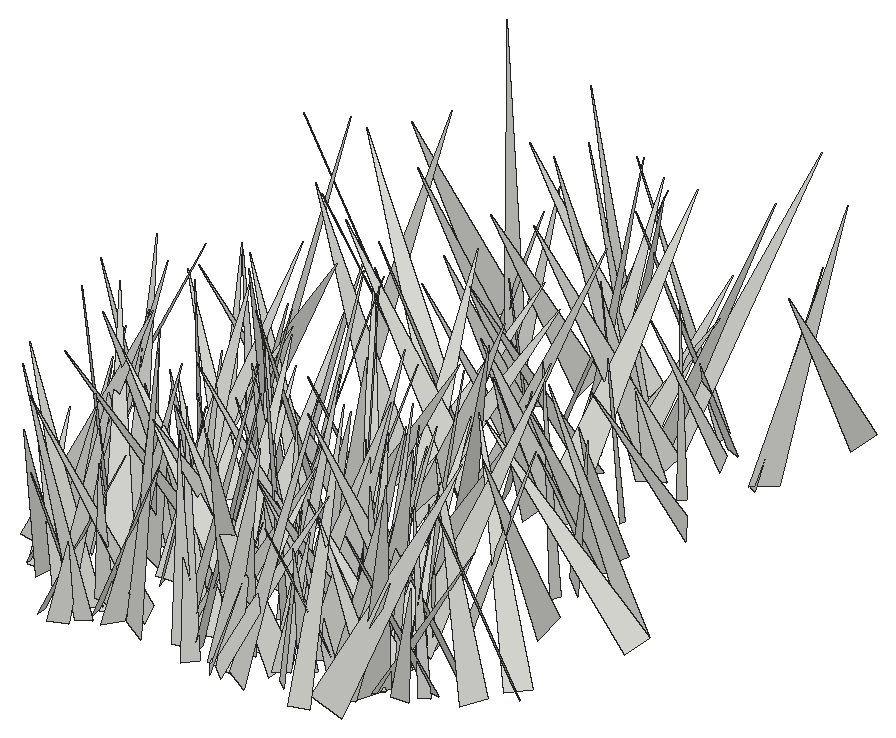
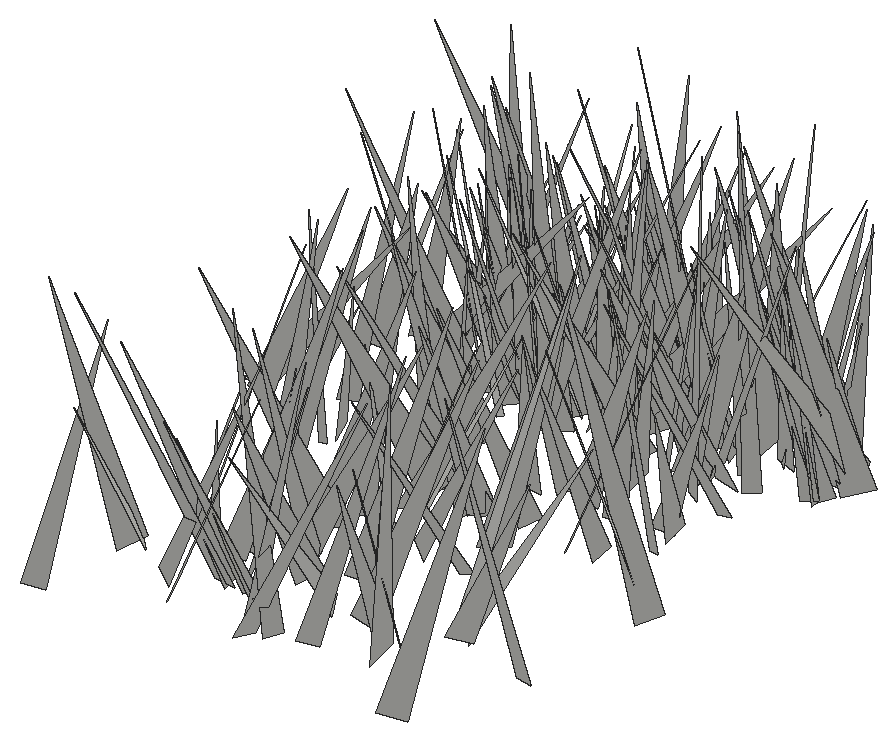
# SketchUp Ruby script. Lengths in inches.
U = 1.inch
M = Sketchup.active_model
def pt(a) = Geom::Point3d.new(a.map { |v| v * U })
def face(e, loops, mat)
  f = e.add_face(loops[0].map { |a| pt(a) })
  loops[1..].each { |l| e.add_face(l.map { |a| pt(a) }).erase! }
  f.material = f.back_material = mat if mat
  f
end
# faces: each face lists its corners as indices into pts; further lists are holes
def faces(e, pts, list, mat = nil) = list.each { |f| face(e, (f[0].is_a?(Array) ? f : [f]).map { |l| l.map { |i| pts[i] } }, mat) }
# xy, xz, yz: faces in a plane at the given z, y or x. An outline is a flat list of corners, or four numbers for a rectangle; further outlines are holes
def ring(l) = l.size == 4 ? [[l[0], l[1]], [l[2], l[1]], [l[2], l[3]], [l[0], l[3]]] : l.each_slice(2).to_a
def flat(e, list, mat, &to3) = list.each { |f| face(e, (f[0].is_a?(Array) ? f : [f]).map { |l| ring(l).map { |u, v| to3.(u, v) } }, mat) }
def xy(e, z, list, mat = nil) = flat(e, list, mat) { |x, y| [x, y, z] }
def xz(e, y, list, mat = nil) = flat(e, list, mat) { |x, z| [x, y, z] }
def yz(e, x, list, mat = nil) = flat(e, list, mat) { |y, z| [x, y, z] }
def lines(e, pts, list) = list.each { |a, b| e.add_line(pt(pts[a]), pt(pts[b])) }
# prism: a flat outline (further loops are holes) pulled along v
def prism(e, loops, v, mat = nil)
  f = face(e, loops, mat); d = Geom::Vector3d.new(v.map { |x| x * U })
  f.pushpull(f.normal.samedirection?(d) ? d.length : -d.length)
end
def box(e, o, s, mat = nil) = prism(e, [[o, [o[0] + s[0], o[1], o[2]], [o[0] + s[0], o[1] + s[1], o[2]], [o[0], o[1] + s[1], o[2]]]], [0, 0, s[2]], mat)
def at(x, y, z, deg = 0) = Geom::Transformation.translation(pt([x, y, z])) * Geom::Transformation.rotation(ORIGIN, Z_AXIS, deg.degrees)
def axes(o, x, y, z) = Geom::Transformation.new([*x, 0, *y, 0, *z, 0, *pt(o).to_a, 1])
def part(name) = M.definitions.add(name)
# library, detail: a bought-in or finely detailed component or shape, given as its bounding box
def library(name, o, s) = part(name).tap { |d| box(d.entities, o, s) }
def detail(e, o, s) = box(e.add_group.entities, o, s)
def put(e, d, t, mat = nil) = e.add_instance(d, t).tap { |i| i.material = mat if mat }
def group(e, t, mat = nil) = e.add_group.tap { |g| g.transformation = t; g.material = mat if mat }.entities
root = M.entities
c1 = part("fur_instance\#9")
p = [[0.8125,0,1.79],[0.67,-0.02,1.48],[0,-0.11,0],[0,0.11,0]]
faces(c1.entities,p,[[0,1,2,3]])
put(root,c1,axes([514.54,139.38,-21.86],[4.00541,-4.88826,1.49079],[-5.10449,-3.91872,0.86522],[-0.24835,1.7057,6.26017]))
put(root,c1,axes([507.39,138.36,-21.66],[-2.16703,-5.16397,2.37315],[-5.48971,1.24499,-2.30381],[-1.47021,2.96275,5.10441]))
put(root,c1,axes([505.36,140.28,-21.86],[-1.78915,-3.44674,0.35763],[-3.41457,1.82215,0.479],[0.59044,0.09337,3.85378]))
put(root,c1,axes([503.11,141.12,-21.86],[4.81338,-2.70132,0.36004],[-2.51999,-4.69011,-1.49931],[-1.0375,-1.14068,5.31205]))
put(root,c1,axes([509.17,140.8,-21.86],[-5.82237,-2.50943,0.01956],[-2.48564,5.77362,0.82736],[0.34528,-0.75212,6.28591]))
put(root,c1,axes([514.33,138.67,-21.86],[3.35941,2.47012,0.56366],[2.52325,-3.34641,-0.37364],[-0.22894,-0.63632,4.15301]))
put(root,c1,axes([507.27,139.99,-21.86],[1.42662,-4.11071,0.89066],[-4.20545,-1.41051,0.22612],[-0.07357,0.91596,4.34535]))
put(root,c1,axes([512.17,139.48,-21.86],[-0.91503,4.79321,2.31879],[5.31141,0.98733,0.05504],[0.37492,-2.28894,4.87946]))
put(root,c1,axes([513.125,142.4375,-21.86],[6.38764,-4.10189,0.26345],[-3.90919,-6.21298,-1.95294],[-1.27011,-1.50671,7.33577]))
put(root,c1,axes([505.22,138.04,-21.86],[4.04294,1.47662,0.10602],[1.40514,-3.92456,1.07725],[-0.46609,0.97696,4.16717]))
put(root,c1,axes([514.49,138.9,-21.86],[3.25743,4.86298,0.41292],[4.6269,-2.91916,-2.12138],[1.55271,-1.50328,5.4552]))
put(root,c1,axes([514.69,140.74,-21.86],[1.67883,-4.20753,0.33675],[-4.18563,-1.61266,0.71764],[0.54516,0.57551,4.47289]))
put(root,c1,axes([516.81,140.66,-21.86],[-6.87538,0.87455,0.95023],[1.06547,6.75006,1.49673],[0.72976,-1.61573,6.76724]))
put(root,c1,axes([507.15,139.64,-21.86],[4.62251,0.92588,0.22465],[0.9419,-4.60847,-0.38752],[-0.14333,-0.42437,4.69837]))
put(root,c1,axes([506.65,139.62,-21.86],[0.94645,-5.69848,3.07489],[-6.04954,-1.88624,-1.63358],[-2.30884,2.60631,5.54074]))
put(root,c1,axes([521.48,141.45,-21.86],[6.44633,-3.37101,0.63256],[-3.2949,-6.46051,-0.8512],[-0.95262,-0.46602,7.22457]))
put(root,c1,axes([509.54,139.25,-21.86],[3.62939,6.32437,2.66269],[6.74766,-3.83695,-0.08396],[-1.24771,-2.35377,7.2913]))
put(root,c1,axes([511.83,140,-21.66],[6.05057,5.41917,1.99571],[5.77348,-5.74186,-1.9125],[-0.1309,-2.76104,7.89425]))
put(root,c1,axes([517.85,143.03,-21.86],[-3.26721,-5.06008,0.08616],[-4.54982,2.98181,2.58736],[2.21606,-1.33826,5.43917]))
put(root,c1,axes([520.91,140.15,-21.86],[3.23817,-2.36152,0.30304],[-2.37388,-3.16317,0.7165],[0.18248,0.75624,3.94324]))
put(root,c1,axes([518.08,140.97,-21.86],[3.30583,-2.31707,0.74955],[-2.21165,-3.38553,-0.71128],[-1.01942,-0.16893,3.97384]))
put(root,c1,axes([520.55,139.21,-21.86],[2.77972,-6.83526,2.99642],[-7.05556,-1.36449,3.4327],[2.43278,3.85274,6.53179]))
put(root,c1,axes([515.93,138.5625,-21.86],[3.6487,6.36792,1.23917],[6.47764,-3.65398,-0.29593],[-0.35515,-1.22351,7.3332]))
put(root,c1,axes([513.45,138.37,-21.66],[-5.70107,0.73605,0.76728],[0.48907,5.53142,-1.67238],[0.94409,1.57933,5.49974]))
put(root,c1,axes([508.53,139,-21.66],[6.30569,-0.68619,2.05979],[-1.17683,-6.39727,1.4715],[-1.82446,1.75482,6.16987]))
put(root,c1,axes([517.73,139.54,-21.86],[2.40724,3.27999,1.19788],[3.2967,-2.61439,0.53362],[-1.15108,-0.62824,4.03341]))
put(root,c1,axes([505.1875,139.44,-21.86],[-4.26519,0.30143,0.24037],[0.24291,4.17451,-0.92459],[0.29939,0.9072,4.17466]))
put(root,c1,axes([511.37,140.84,-21.86],[3.22787,2.03353,0.24614],[1.96333,-2.94045,-1.45397],[0.58408,-1.35405,3.52709]))
put(root,c1,axes([517,140.42,-21.86],[2.68991,-2.47286,1.2383],[-2.72716,-2.65872,0.6147],[-0.45937,1.30393,3.60178]))
put(root,c1,axes([506.62,137.47,-21.66],[-6.46453,1.71895,1.7422],[0.79023,6.12289,-3.109],[2.31637,2.70842,5.92275]))
put(root,c1,axes([522.67,141.78,-21.86],[1.50872,-3.69838,0.31644],[-3.67115,-1.43625,0.71715],[0.54852,0.55997,3.92937]))
put(root,c1,axes([515.29,141.26,-21.66],[-6.72983,3.60579,0.05795],[3.45053,6.40273,2.3226],[-1.04828,-2.07339,7.27309]))
put(root,c1,axes([503.29,141.59,-21.66],[0.14432,-5.01914,1.5992],[-4.96199,0.40759,1.72702],[1.76858,1.55311,4.71487]))
put(root,c1,axes([519.85,138.08,-21.66],[1.21236,6.8418,0.01969],[6.58716,-1.17263,1.87473],[-1.84929,0.30844,6.6907]))
put(root,c1,axes([514.65,139.02,-21.86],[-0.90144,4.87523,0.09791],[4.65666,0.89022,-1.45364],[1.44671,0.1723,4.73998]))
put(root,c1,axes([512.85,139.67,-21.86],[5.6278,2.51424,1.57514],[2.22036,-5.80941,1.3399],[-1.96786,0.63554,6.01649]))
put(root,c1,axes([519.99,141.29,-21.86],[-0.77592,-4.15559,2.31409],[-4.39268,1.52537,1.26634],[1.82437,1.90534,4.03328]))
put(root,c1,axes([505.83,142.6,-21.86],[-5.15951,-5.90719,2.53837],[-5.9684,5.61072,0.92562],[2.3909,1.25844,7.78837]))
put(root,c1,axes([521.45,141.6,-21.86],[-1.9475,3.70978,1.3462],[3.85912,1.47603,1.51527],[-0.82582,-1.85103,3.9063]))
put(root,c1,axes([523.49,143.12,-21.86],[-1.6318,-4.41068,0.10105],[-4.3461,1.58854,-0.8456],[-0.75876,0.38671,4.62621]))
put(root,c1,axes([507.91,140.22,-21.86],[-4.53452,6.13099,1.20513],[6.2123,4.58336,0.05748],[0.66981,-1.00349,7.62546]))
put(root,c1,axes([511.8,141.28,-21.86],[-4.39525,1.44739,0.73649],[1.42922,4.45652,-0.22883],[0.77116,-0.01,4.62177]))
put(root,c1,axes([513.48,143.48,-21.66],[-2.19661,-7.3796,0.4517],[-6.30745,1.62463,-4.13089],[-3.85727,1.54587,6.49764]))
put(root,c1,axes([512.29,145.55,-21.66],[6.08199,-2.63161,2.26399],[-1.13407,-5.82276,-3.72169],[-3.281,-2.8656,5.48316]))
put(root,c1,axes([502.46,141.11,-21.86],[-0.72601,3.76819,0.7458],[3.80081,0.81458,-0.41575],[0.55615,-0.64789,3.8149]))
put(root,c1,axes([518.82,141.81,-21.86],[0.00954,3.59248,1.3323],[3.47361,-0.5704,1.51319],[-1.6171,-1.20405,3.25826]))
put(root,c1,axes([520.97,142.79,-21.86],[-2.91318,-3.12111,0.33199],[-3.12229,2.8354,-0.74159],[-0.32068,0.74655,4.20452]))
put(root,c1,axes([519.35,141.88,-21.86],[6.46627,-2.11143,1.67342],[-2.36842,-6.52888,0.91405],[-1.28416,1.40953,6.74057]))
put(root,c1,axes([501.25,142.79,-21.86],[3.50419,-7.42751,1.71848],[-7.22357,-2.63012,3.36199],[2.43745,2.88357,7.49295]))
put(root,c1,axes([518.51,144.58,-21.66],[0.56796,-5.36738,0.34113],[-5.01782,-0.65229,-1.90884],[-1.93561,0.11605,5.04853]))
put(root,c1,axes([521.62,143.34,-21.66],[-4.01783,2.35497,0.3103],[2.27352,3.63609,1.84258],[-0.68795,-1.73727,4.27712]))
put(root,c1,axes([521.55,141.67,-21.86],[4.38555,-0.36882,0.03632],[-0.36139,-4.16033,1.38975],[0.08213,1.3878,4.17584]))
put(root,c1,axes([505.02,145.68,-21.86],[-1.84089,-7.99139,1.4242],[-7.16502,2.28604,3.56596],[3.81486,0.4373,7.3848]))
put(root,c1,axes([504.19,141.93,-21.86],[3.861,5.57007,1.34937],[5.71182,-3.87341,-0.35436],[-0.47072,-1.31331,6.76812]))
put(root,c1,axes([516.91,145.04,-21.66],[-7.35388,-1.92649,0.06127],[-1.88282,7.23164,1.39751],[0.41243,-1.33667,7.47248]))
put(root,c1,axes([513.2,140.84,-21.66],[-3.83392,6.10516,1.11787],[5.9137,3.99214,-1.52073],[1.88436,-0.10697,7.04694]))
put(root,c1,axes([511.68,143.87,-21.86],[2.07826,-5.21506,0.82935],[-4.82149,-1.51054,2.58366],[2.15357,1.65083,4.98405]))
put(root,c1,axes([516.4,144.94,-21.86],[-2.66612,-3.28273,0.28859],[-3.19335,2.6653,0.81637],[0.81369,-0.29607,4.14946]))
put(root,c1,axes([520.8125,145.92,-21.66],[-7.04471,-1.4589,1.32068],[-0.96261,6.83613,2.41686],[1.71638,-2.15394,6.77607]))
put(root,c1,axes([516.34,141.43,-21.86],[2.11808,6.39246,0.96016],[6.39192,-2.22182,0.69185],[-0.96378,-0.68681,6.6986]))
put(root,c1,axes([521.43,143.65,-21.86],[4.62058,2.87983,1.50344],[3.15499,-4.60106,-0.88304],[-0.77446,-1.56215,5.37246]))
put(root,c1,axes([520.48,142.05,-21.66],[-5.01766,-1.40088,1.70753],[-1.93126,4.83928,-1.7049],[1.07162,2.16194,4.92267]))
put(root,c1,axes([511.08,141.1,-21.66],[-5.97598,0.81352,1.54005],[0.17172,5.75229,-2.37225],[1.73323,2.235,5.54496]))
put(root,c1,axes([509.61,144.42,-21.86],[-0.73911,-5.79285,1.55471],[-5.99778,0.70592,-0.22109],[-0.03032,1.57006,5.83563]))
put(root,c1,axes([515.45,142.72,-21.86],[-6.49961,-2.89491,2.26898],[-3.37847,6.5202,-1.35892],[1.4542,2.20912,6.98418]))
put(root,c1,axes([502.66,142.99,-21.86],[0.08637,4.97569,1.67082],[5.15736,0.22998,-0.95146],[0.97504,-1.65717,4.88463]))
put(root,c1,axes([520.44,142.45,-21.86],[-0.17119,5.69768,1.30234],[5.83131,0.07859,0.42267],[-0.39436,-1.31119,5.68456]))
put(root,c1,axes([525.44,143.59,-21.86],[-5.24229,2.67543,1.59997],[2.88849,5.34612,0.52444],[1.17239,-1.20849,5.86212]))
put(root,c1,axes([517.9375,142.125,-21.66],[7.25129,-2.23194,2.73946],[-2.93898,-7.28136,1.84704],[-1.96177,2.6585,7.35875]))
put(root,c1,axes([515.91,143.38,-21.66],[3.27115,-5.93629,2.22387],[-6.24966,-2.60094,2.25],[1.06155,2.98013,6.39355]))
put(root,c1,axes([507.83,146.5625,-21.66],[3.07442,-7.15508,0.96712],[-6.88437,-3.22185,-1.95131],[-2.1762,0.08396,7.5392]))
put(root,c1,axes([526.37,145.44,-21.86],[-3.22391,-4.50813,0.36238],[-4.51102,3.23719,0.13952],[0.32445,0.21334,5.54053]))
put(root,c1,axes([505.39,142.76,-21.86],[0.59003,4.76484,1.13067],[4.77949,-0.80843,0.91275],[-1.06703,-0.9864,4.71367]))
put(root,c1,axes([507.69,143.67,-21.86],[4.51759,1.55237,1.02195],[1.60919,-4.61101,-0.10928],[-0.92991,-0.4377,4.77562]))
put(root,c1,axes([506.14,144.69,-21.86],[-0.90647,-5.11686,1.80724],[-5.12934,1.40604,1.40817],[1.7715,1.45288,5.00209]))
put(root,c1,axes([502.05,144.19,-21.86],[2.80159,-3.67069,0.58517],[-3.61323,-2.51742,1.50747],[0.87232,1.36159,4.36468]))
put(root,c1,axes([502.2,144.55,-21.86],[5.07227,1.20948,1.05659],[1.39553,-5.05165,-0.91676],[-0.7948,-1.15114,5.13326]))
put(root,c1,axes([518.58,145.3,-21.86],[1.54796,-4.76639,0.70367],[-4.81569,-1.50748,0.38266],[0.1508,0.78667,4.99682]))
put(root,c1,axes([508.61,144.37,-21.86],[-1.858,-4.3991,1.45242],[-4.62148,1.65138,-0.9103],[-0.32175,1.68364,4.68782]))
put(root,c1,axes([523.68,142.29,-21.66],[-4.92435,-0.05312,0.24709],[-0.15186,4.47527,-2.06445],[0.20202,2.06935,4.47102]))
put(root,c1,axes([502.33,144.95,-21.66],[0.76926,-4.66703,1.07076],[-4.59745,-0.41678,1.48633],[1.33832,1.25083,4.49041]))
put(root,c1,axes([511.6875,141.59,-21.86],[4.83042,2.64277,1.00625],[2.0268,-4.62442,2.4159],[-1.97202,1.72053,4.9478]))
put(root,c1,axes([515.22,144.71,-21.86],[5.25974,-3.61511,1.15521],[-3.73911,-5.27428,0.51907],[-0.65007,1.0869,6.36116]))
put(root,c1,axes([518.4,146.09,-21.86],[4.17782,-5.39394,0.17375],[-5.37681,-4.14138,0.71959],[0.46328,0.57738,6.78461]))
put(root,c1,axes([514.27,144.42,-21.86],[-2.98009,3.50221,2.17702],[3.82104,3.35523,-0.16707],[1.55067,-1.53712,4.59549]))
put(root,c1,axes([506.98,141.87,-21.86],[-7.79963,1.89477,1.60693],[1.33324,7.65978,-2.56065],[2.09639,2.17814,7.60707]))
put(root,c1,axes([519.84,143.05,-21.86],[5.12063,-0.00436,1.95562],[-0.62511,-5.19742,1.62522],[-1.85303,1.74129,4.85588]))
put(root,c1,axes([521.23,143.04,-21.66],[2.56304,5.03632,1.18387],[4.82189,-2.80423,1.49027],[-1.87495,-0.32715,5.45094]))
put(root,c1,axes([508.32,143.6,-21.66],[-2.56408,6.91655,2.55207],[6.94878,3.17004,-1.60986],[2.46298,-1.74312,7.19872]))
put(root,c1,axes([502.9,144.16,-21.86],[4.61104,6.12434,1.67223],[6.3457,-4.50796,-0.9879],[-0.18966,-1.93296,7.60219]))
put(root,c1,axes([517.85,145.4375,-21.86],[2.0151,-5.02328,1.60572],[-5.27188,-1.87389,0.75376],[0.13771,1.76848,5.35965]))
put(root,c1,axes([514.32,145.36,-21.86],[-5.21279,-1.15752,0.50027],[-1.17064,5.23306,-0.0898],[0.46875,0.19648,5.33901]))
put(root,c1,axes([524.03,144.51,-21.66],[-5.38862,-5.55187,0.24968],[-4.68183,4.34761,-4.37054],[-2.99434,3.19341,6.38427]))
put(root,c1,axes([512.28,146.62,-21.86],[1.37866,-6.43403,1.32521],[-6.55871,-1.42426,-0.09169],[-0.36909,1.27608,6.57944]))
put(root,c1,axes([515.28,146.72,-21.86],[1.49707,-8.01218,1.60299],[-8.01526,-1.12338,1.87068],[1.58751,1.88383,7.93327]))
put(root,c1,axes([501.97,141.48,-21.86],[7.75154,3.11882,0.30174],[2.75499,-7.16733,3.30818],[-1.4927,2.96765,7.67264]))
put(root,c1,axes([507.35,145.24,-21.86],[-7.20158,-1.52489,0.67202],[-1.60184,7.15641,-0.92717],[0.45935,1.04894,7.30263]))
put(root,c1,axes([509.08,146.75,-21.86],[-3.29784,-3.61715,1.25797],[-3.53735,3.51322,0.8285],[1.46745,0.33986,4.82422]))
put(root,c1,axes([511.72,142.97,-21.86],[-3.94963,4.34285,0.40783],[4.0226,3.83915,-1.92507],[1.68683,1.01332,5.54563]))
put(root,c1,axes([516.1875,146.62,-21.86],[-4.11377,-6.51171,1.45116],[-6.65439,3.88319,-1.43913],[-0.47668,1.98739,7.56666]))
put(root,c1,axes([517.89,147.5,-21.66],[5.66121,2.03663,0.41958],[1.99596,-4.98096,-2.75306],[0.58316,-2.72311,5.34956]))
put(root,c1,axes([521.08,143.31,-21.66],[-3.49002,4.97532,0.38419],[4.70613,3.43753,-1.76559],[1.65943,0.71499,5.81522]))
put(root,c1,axes([510.06,144.0625,-21.86],[6.46332,2.41268,1.62775],[2.03661,-6.58136,1.66821],[-2.07914,1.05343,6.69422]))
put(root,c1,axes([521,144.88,-21.86],[4.76999,5.26227,1.90717],[5.37132,-5.00824,0.38463],[-1.57405,-1.14351,7.09199]))
put(root,c1,axes([518.73,144.59,-21.86],[2.68207,4.86571,0.6841],[4.89534,-2.71316,0.10499],[-0.42283,-0.54794,5.55496]))
put(root,c1,axes([511.86,146.07,-21.86],[-1.05184,5.80364,2.59591],[6.34975,1.09094,0.13387],[0.3189,-2.57972,5.89666]))
put(root,c1,axes([506.64,147.87,-21.66],[-4.19902,-6.23031,2.61813],[-6.01537,4.8505,1.89504],[3.08005,0.97931,7.27031]))
put(root,c1,axes([515.68,144.46,-21.86],[5.3948,4.35682,0.5893],[4.31887,-5.42625,0.57994],[-0.82254,0.08385,6.9101]))
put(root,c1,axes([521.04,146.4375,-21.86],[3.01328,1.01562,1.71575],[1.06477,-3.44849,0.1713],[-1.68569,-0.36275,3.17522]))
put(root,c1,axes([522.18,146.57,-21.86],[4.42305,4.26534,0.99754],[4.37397,-4.22348,-1.33498],[0.23791,-1.64944,5.99786]))
put(root,c1,axes([526.31,145.68,-21.86],[-2.5947,5.83184,0.30944],[5.66182,2.42897,1.69778],[-1.43174,-0.96349,6.15308]))
put(root,c1,axes([507.72,146.8125,-21.86],[-2.80157,3.07223,0.58027],[3.12461,2.72376,0.66487],[-0.11008,-0.87559,4.10431]))
put(root,c1,axes([520.29,146.02,-21.86],[1.6055,7.88479,1.47704],[7.72527,-1.11383,-2.45126],[2.16141,-1.87581,7.66412]))
put(root,c1,axes([524.07,150.64,-21.66],[6.25747,-1.85529,1.59771],[-1.00282,-5.94215,-2.97253],[-2.23363,-2.52972,5.81052]))
put(root,c1,axes([516.98,145.93,-21.66],[5.31118,5.11176,2.74997],[4.78098,-5.96627,1.85658],[-3.29161,-0.41778,7.13385]))
put(root,c1,axes([518.46,145.68,-21.66],[1.86893,4.92203,0.04113],[4.36091,-1.67616,2.42774],[-2.28266,0.8277,4.67176]))
put(root,c1,axes([506.34,145.82,-21.86],[2.50136,7.65725,0.1478],[7.63522,-2.48107,-0.67805],[0.59891,-0.35058,8.02686]))
put(root,c1,axes([512.02,145.51,-21.66],[6.2923,4.31715,0.79405],[3.75537,-6.01297,2.93303],[-2.27277,2.01685,7.04472]))
put(root,c1,axes([507.96,151.76,-21.66],[-1.88375,-7.99896,1.23534],[-7.80751,2.13018,1.88761],[2.13359,0.73274,7.99805]))
put(root,c1,axes([512.45,146.66,-21.66],[3.92721,6.27569,0.86047],[6.07775,-4.01843,1.56873],[-1.78486,0.12492,7.23508]))
put(root,c1,axes([510.55,146.5,-21.66],[-4.56425,4.1816,0.8559],[3.58274,4.43445,-2.55936],[2.31998,1.37862,5.63629]))
put(root,c1,axes([504.38,148.39,-21.66],[2.28513,5.39499,0.34939],[5.12885,-2.04337,-1.99232],[1.70965,-1.08097,5.50984]))
put(root,c1,axes([516.94,149.92,-21.66],[4.74645,-3.63152,0.20608],[-3.44873,-4.38539,2.15263],[1.15614,1.82746,5.57521]))
put(root,c1,axes([509.33,148.41,-21.66],[-6.71,0.21588,0.88951],[-0.0468,6.49159,-1.92847],[0.91413,1.91692,6.43053]))
put(root,c1,axes([511.33,151.13,-21.66],[1.52564,-3.34819,0.07276],[-3.07421,-1.36842,1.48995],[1.32851,0.67846,3.36423]))
put(root,c1,axes([528.11,151.91,-21.66],[-5.02457,3.67244,0.21301],[3.24783,4.25941,3.17608],[-1.72736,-2.67378,5.35216]))
put(root,c1,axes([510.14,151.2,-21.66],[-1.88222,6.06948,1.49765],[6.0067,1.32242,2.18977],[-1.73238,-2.00921,5.96542]))
put(root,c1,axes([504.8,152.93,-21.66],[3.94876,4.2171,2.00571],[4.64379,-3.26946,-2.26834],[0.4919,-2.98768,5.31331]))
put(root,c1,axes([508.03,155.12,-21.66],[-6.16351,-3.9605,0.27898],[-3.73191,5.95492,2.08903],[1.35509,-1.6142,7.02213]))
put(root,c1,axes([505.7,151.17,-21.66],[-2.49681,4.68547,0.3153],[4.52882,2.308,1.56527],[-1.24213,-1.0033,5.07323]))
put(root,c1,axes([527.52,152.65,-21.66],[-0.80032,5.57612,2.90873],[5.9333,-0.30294,2.21326],[-2.08561,-3.00158,5.18026]))
put(root,c1,axes([515.9,154.59,-21.66],[7.05622,-1.23215,0.51957],[-1.10047,-6.93599,-1.50315],[-0.75967,-1.39725,7.0035]))
put(root,c1,axes([522.54,154.35,-21.66],[-1.98967,-4.65459,1.69235],[-4.24096,2.54317,2.00863],[2.55803,0.59592,4.64644]))
put(root,c1,axes([505.1,151.02,-21.66],[-5.60466,1.1961,0.32776],[0.92969,5.05609,-2.5538],[0.82084,2.4404,5.13039]))
put(root,c1,axes([522.93,156.31,-21.66],[2.61621,-5.42084,0.25429],[-5.22177,-2.59146,-1.52055],[-1.47757,-0.43991,5.82391]))
put(root,c1,axes([524.6,154.33,-21.66],[-1.27388,-3.61865,0.59779],[-3.46584,0.98064,-1.44951],[-1.19998,1.0092,3.55195]))
put(root,c1,axes([512.8125,151.85,-21.66],[-0.78819,5.89997,0.04998],[5.7265,0.75282,1.4401],[-1.42105,-0.23877,5.77555]))
put(root,c1,axes([510.75,154.23,-21.66],[4.20762,-3.32651,0.12048],[-3.15177,-3.91891,1.86887],[1.07075,1.53645,5.02763]))
put(root,c1,axes([522.55,152.99,-21.66],[-5.22043,-0.84385,1.05571],[-1.17009,4.93002,-1.84535],[0.67639,2.01552,4.95577]))
put(root,c1,axes([522.61,157.27,-21.66],[4.609,-3.3139,0.05026],[-3.15306,-4.41083,-1.68231],[-1.0211,-1.33793,5.42168]))
put(root,c1,axes([513.3125,155.19,-21.66],[4.4628,-4.8312,0.78242],[-4.8199,-4.15484,1.83716],[0.84924,1.80724,6.31521]))
put(root,c1,axes([515.79,156.54,-21.66],[-7.5943,2.08618,0.38061],[2.11361,7.33132,1.9887],[-0.17228,-2.01745,7.62041]))
put(root,c1,axes([501.11,157.83,-21.66],[2.01455,-7.63294,0.11302],[-6.59973,-1.68273,3.99311],[3.83642,1.11337,6.80994]))
put(root,c1,axes([510.69,156.93,-21.66],[-6.83352,3.26319,2.339],[3.80782,6.73136,1.73366],[1.27275,-2.61852,7.37155]))
put(root,c1,axes([506.48,154.53,-21.66],[5.33264,0.16428,1.51785],[-0.27785,-5.31816,1.55174],[-1.50122,1.56784,5.10452]))
put(root,c1,axes([517.03,158.35,-21.66],[4.74802,-2.11154,0.82126],[-1.70244,-4.58339,-1.94189],[-1.49491,-1.48682,4.81989]))
put(root,c1,axes([512.66,154.83,-21.66],[1.506,6.6666,0.93752],[6.04421,-0.91584,-3.19677],[2.9648,-1.51928,6.04088]))
put(root,c1,axes([515.3125,155.98,-21.66],[-5.46904,-3.01802,0.13387],[-2.92547,5.22183,-1.79189],[-0.75368,1.63119,5.98398]))
put(root,c1,axes([518.75,158.54,-21.66],[3.32641,-4.64571,1.36805],[-4.19977,-3.59363,-1.99171],[-2.41165,-0.14974,5.35544]))
put(root,c1,axes([512.97,154.89,-21.66],[-3.56356,5.20391,0.71647],[5.00613,3.62664,-1.4419],[1.59144,0.24443,6.14008]))
put(root,c1,axes([515.75,154.59,-21.66],[7.47799,-1.52657,1.95795],[-2.25093,-6.79047,3.30259],[-1.04752,3.69369,6.88067]))
put(root,c1,axes([515.07,158.78,-21.66],[4.19489,0.81761,0.41517],[0.91291,-3.90671,-1.53042],[-0.08632,-1.58339,3.99042]))
put(root,c1,axes([523.16,161.59,-21.66],[-4.76497,-3.93422,0.44703],[-3.2824,4.31602,2.99679],[2.21445,-2.06803,5.40391]))
put(root,c1,axes([503.11,156.14,-21.66],[5.00071,5.94343,0.88428],[5.7504,-5.06729,1.53914],[-1.74336,0.3341,7.61331]))
put(root,c1,axes([513.05,159.3125,-21.66],[-3.40667,-4.88664,0.79026],[-4.79108,3.01371,-2.01797],[-1.2447,1.77411,5.60468]))
put(root,c1,axes([507.74,162.75,-21.66],[-4.53794,-6.8341,0.16977],[-6.57814,4.42074,2.12406],[1.86058,-1.03861,7.92377]))
put(root,c1,axes([512.99,162.21,-21.66],[-4.86193,-2.9811,0.43497],[-2.74592,4.72474,1.68858],[1.2394,-1.22654,5.44739]))
put(root,c1,axes([513.48,163.02,-21.66],[3.27903,-5.74844,0.73311],[-5.41958,-3.34021,-1.9507],[-2.05188,-0.36394,6.32387]))
put(root,c1,axes([516.72,162.96,-21.66],[0.00181,-5.98408,0.19016],[-5.68264,-0.06159,-1.88392],[-1.88493,0.17992,5.67979]))
put(root,c1,axes([510.05,159.64,-21.66],[1.05381,5.0713,0.10966],[4.76326,-0.95083,-1.80217],[1.74396,-0.4674,4.856]))
put(root,c1,axes([520.58,160.26,-21.66],[-5.03149,-1.83162,1.20846],[-2.18082,4.50919,-2.24552],[0.24343,2.5384,4.86091]))
put(root,c1,axes([519.12,165.11,-21.66],[-7.73279,0.49202,2.83462],[1.75633,7.24586,3.53356],[2.27869,-3.91518,6.89581]))
put(root,c1,axes([517.32,160.05,-21.66],[-1.94232,7.80928,1.11049],[7.41359,2.19794,-2.48968],[2.69386,-0.41817,7.65238]))
put(root,c1,axes([519.29,163.93,-21.66],[-0.93338,-7.69941,2.7531],[-7.87622,0.10215,-2.38461],[-2.19672,2.90522,7.38009]))
put(root,c1,axes([506.74,163.71,-21.66],[-5.49378,-4.48735,0.1731],[-4.21573,5.05933,-2.64174],[-1.54724,2.14821,6.58325]))
put(root,c1,axes([510.81,166,-21.66],[0.32689,-6.93131,1.01824],[-6.72809,-0.59471,-1.88835],[-1.95261,0.88881,6.67713]))
put(root,c1,axes([510.66,165.76,-21.66],[-2.98653,-2.99705,1.42564],[-2.58075,3.30304,1.53746],[2.08674,-0.20437,3.94181]))
put(root,c1,axes([521.4,163.46,-21.66],[-4.31752,-0.25034,0.73123],[-0.52227,4.00392,-1.71296],[0.56974,1.77322,3.97108]))
put(root,c1,axes([515.97,163.19,-21.66],[6.62272,2.03005,2.53711],[1.31072,-6.93962,2.13125],[-2.97322,1.46257,6.59085]))
put(root,c1,axes([520.82,167.17,-21.66],[-4.32918,-1.79601,0.73607],[-1.48596,4.22424,1.56749],[1.24875,-1.19977,4.41706]))
put(root,c1,axes([506.58,164.57,-21.66],[-3.94655,4.7323,0.06828],[4.56087,3.77904,1.70056],[-1.26405,-1.13963,5.92267]))
put(root,c1,axes([511.64,169.02,-21.66],[6.11084,-2.63091,1.80363],[-1.49433,-5.80472,-3.40432],[-2.81811,-2.62692,5.71618]))
put(root,c1,axes([501.99,165.72,-21.66],[3.4737,5.90005,1.74495],[6.11319,-3.08303,-1.74525],[0.69596,-2.36778,6.62052]))
put(root,c1,axes([515.35,164.23,-21.66],[-5.11664,3.91829,0.85035],[3.38571,4.96082,-2.48663],[2.14782,1.51438,5.94556]))
put(root,c1,axes([517.5,165.8125,-21.66],[-6.96753,-1.64469,0.65915],[-1.76863,6.61713,-2.18437],[0.10697,2.27915,6.81763]))
put(root,c1,axes([520.47,168.26,-21.66],[-3.35511,-5.27651,0.83113],[-5.27558,3.11951,-1.49198],[-0.83701,1.48869,6.07225]))
put(root,c1,axes([513.3125,169.42,-21.66],[7.4678,0.08394,0.57516],[0.2355,-7.21321,-2.00499],[-0.53141,-2.01703,7.1941]))
put(root,c1,axes([515.43,168,-21.66],[2.92691,3.10527,0.26779],[2.82947,-2.4932,-2.01476],[1.3071,-1.55642,3.76168]))
put(root,c1,axes([516.48,167.02,-21.66],[0.2906,4.64928,0.9365],[4.41539,0.07727,-1.75374],[1.73123,-0.9775,4.31562]))
put(root,c1,axes([506.51,168.35,-21.66],[3.8282,2.91024,0.83789],[3.01788,-3.55309,-1.44728],[0.25298,-1.65308,4.58585]))
put(root,c1,axes([509.3125,166.53,-21.66],[4.39596,-0.31282,2.17467],[-1.10489,-4.51925,1.5834],[-1.89902,1.90528,4.11281]))
put(root,c1,axes([517.9,166.39,-21.66],[6.72656,-0.08852,1.07497],[-0.40385,-6.50233,1.99163],[-1.00015,2.03024,6.42556]))
put(root,c1,axes([523.47,166.77,-21.66],[6.60662,-2.19065,2.41659],[-2.83754,-6.55209,1.81792],[-1.6085,2.56075,6.71874]))
put(root,c1,axes([512.93,165.54,-21.66],[4.98815,3.01806,0.37753],[2.59556,-4.60182,2.49383],[-1.58564,1.9615,5.26983]))
put(root,c1,axes([515.75,167.67,-21.66],[-7.81157,-0.92448,1.21309],[-1.13809,7.74743,-1.42443],[1.01538,1.5715,7.73604]))
put(root,c1,axes([523.26,166.2,-21.66],[3.56764,3.88458,0.34534],[3.52617,-3.41301,1.96335],[-1.66594,1.09483,4.89523]))
put(root,c1,axes([514.37,170.15,-21.66],[-6.85321,0.30824,0.48855],[0.41589,6.6696,1.62593],[0.40091,-1.64973,6.66467]))
put(root,c1,axes([504.55,171.89,-21.66],[4.75153,-4.99406,0.9078],[-4.47168,-4.70683,-2.48828],[-2.40183,-1.11663,6.42854]))
put(root,c1,axes([518.02,166.96,-21.66],[3.14457,7.68443,0.45621],[7.56933,-2.99688,-1.69436],[1.40136,-1.05601,8.12822]))
put(root,c1,axes([508.48,167.77,-21.66],[-8.04005,-0.21045,2.18635],[-0.63833,8.16213,-1.56173],[2.10165,1.67397,7.88972]))
put(root,c1,axes([524.47,172.58,-21.66],[5.34512,-3.23236,0.64666],[-2.65449,-4.95104,-2.80671],[-1.95449,-2.11559,5.5804]))
put(root,c1,axes([519.36,169.07,-21.66],[-6.43064,-2.17008,0.24743],[-2.17262,6.27662,-1.4168],[-0.22404,1.42068,6.6374]))
